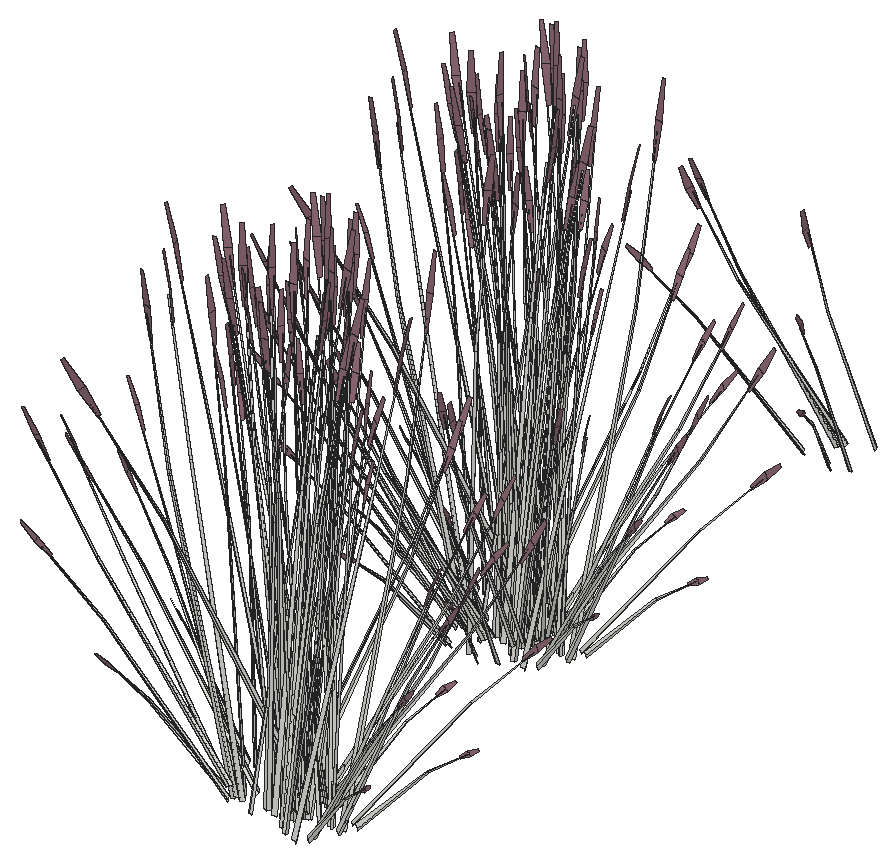
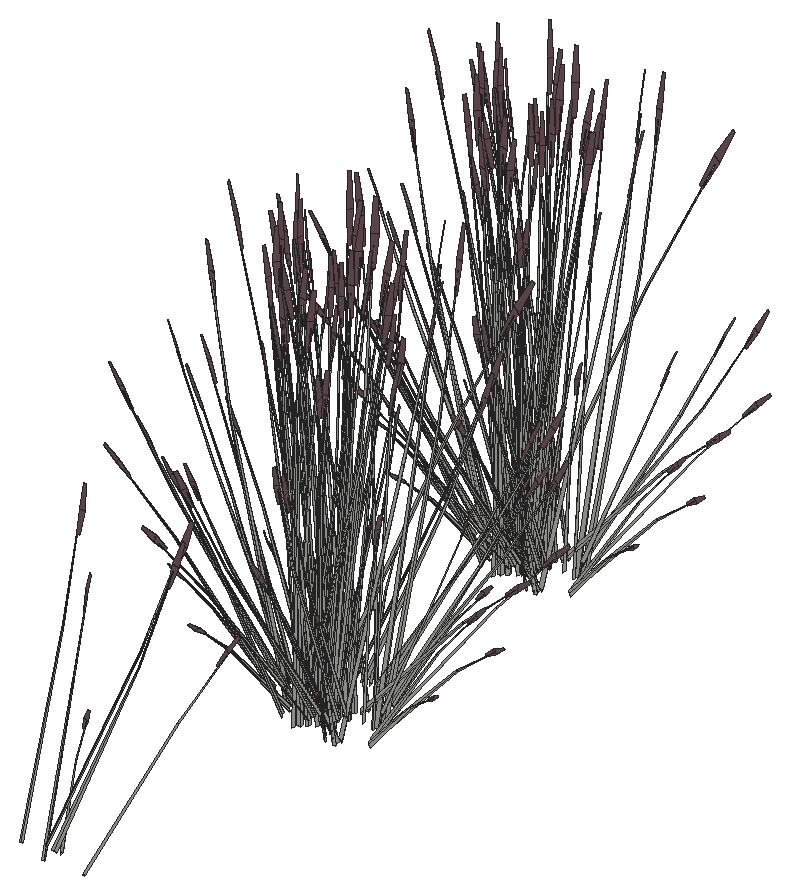
# SketchUp Ruby script. Lengths in inches.
U = 1.inch
M = Sketchup.active_model
def pt(a) = Geom::Point3d.new(a.map { |v| v * U })
def face(e, loops, mat)
  f = e.add_face(loops[0].map { |a| pt(a) })
  loops[1..].each { |l| e.add_face(l.map { |a| pt(a) }).erase! }
  f.material = f.back_material = mat if mat
  f
end
# faces: each face lists its corners as indices into pts; further lists are holes
def faces(e, pts, list, mat = nil) = list.each { |f| face(e, (f[0].is_a?(Array) ? f : [f]).map { |l| l.map { |i| pts[i] } }, mat) }
# xy, xz, yz: faces in a plane at the given z, y or x. An outline is a flat list of corners, or four numbers for a rectangle; further outlines are holes
def ring(l) = l.size == 4 ? [[l[0], l[1]], [l[2], l[1]], [l[2], l[3]], [l[0], l[3]]] : l.each_slice(2).to_a
def flat(e, list, mat, &to3) = list.each { |f| face(e, (f[0].is_a?(Array) ? f : [f]).map { |l| ring(l).map { |u, v| to3.(u, v) } }, mat) }
def xy(e, z, list, mat = nil) = flat(e, list, mat) { |x, y| [x, y, z] }
def xz(e, y, list, mat = nil) = flat(e, list, mat) { |x, z| [x, y, z] }
def yz(e, x, list, mat = nil) = flat(e, list, mat) { |y, z| [x, y, z] }
def lines(e, pts, list) = list.each { |a, b| e.add_line(pt(pts[a]), pt(pts[b])) }
# prism: a flat outline (further loops are holes) pulled along v
def prism(e, loops, v, mat = nil)
  f = face(e, loops, mat); d = Geom::Vector3d.new(v.map { |x| x * U })
  f.pushpull(f.normal.samedirection?(d) ? d.length : -d.length)
end
def box(e, o, s, mat = nil) = prism(e, [[o, [o[0] + s[0], o[1], o[2]], [o[0] + s[0], o[1] + s[1], o[2]], [o[0], o[1] + s[1], o[2]]]], [0, 0, s[2]], mat)
def at(x, y, z, deg = 0) = Geom::Transformation.translation(pt([x, y, z])) * Geom::Transformation.rotation(ORIGIN, Z_AXIS, deg.degrees)
def axes(o, x, y, z) = Geom::Transformation.new([*x, 0, *y, 0, *z, 0, *pt(o).to_a, 1])
def part(name) = M.definitions.add(name)
# library, detail: a bought-in or finely detailed component or shape, given as its bounding box
def library(name, o, s) = part(name).tap { |d| box(d.entities, o, s) }
def detail(e, o, s) = box(e.add_group.entities, o, s)
def put(e, d, t, mat = nil) = e.add_instance(d, t).tap { |i| i.material = mat if mat }
def group(e, t, mat = nil) = e.add_group.tap { |g| g.transformation = t; g.material = mat if mat }.entities
root = M.entities
M.materials.add("LightPink_Translucent").color = [144, 107, 117]
c1 = part("blade")
p = [[2.15,0.21,22],[0,0.17,0],[0.09,0.45,0],[2.18,0.31,22],[2.29,0.31,22],[0.38,0.45,0],
  [2.48,0.24,33],[2.49,0.24,33],[2.48,0.22,33]]
faces(c1.entities,p,[[0,1,2,3],[4,5,2,3],[6,3,4,7],[8,0,3,6]])
c2 = part("seeds")
p = [[0.3,-0.1,1.38],[-0.01,-0.03,1.59],[-0.01,-0.03,0.03],[0.14,-0.07,-0.07],[0.29,-0.03,3],[0.15,0.01,3.11]]
faces(c2.entities,p,[[0,1,2,3],[1,0,4,5]],"LightPink_Translucent")
c3 = part("blade with seeds")
put(c3.entities,c1,at(0,0,0))
put(c3.entities,c2,axes([2.4,0.25,30.99],[1.5799,-0.05474,1.17369],[-0.12525,1.92788,0.29478],[-0.07173,-0.02425,1.56792]))
put(root,c3,axes([53.92,557.8,45.33],[1.05902,0.41762,1.51261],[-1.03748,0.89969,0.59816],[-0.46471,-0.53324,1.26806]))
put(root,c3,axes([59,553.64,44.59],[-0.4378,-0.03068,1.43002],[-0.44851,-0.8229,-0.30754],[0.53783,-0.23279,0.61141]))
put(root,c3,axes([59.51,552.125,44.77],[-0.40819,0.5272,1.1486],[-0.35086,-0.70831,0.84392],[0.33713,-0.17749,0.25299]))
put(root,c3,axes([48.05,555.7,44.375],[-1.53239,0,0],[0,-1.1575,-0.51607],[0,-0.26363,1.63711]))
put(root,c3,axes([48.31,553.63,44.59],[0.23927,0.28834,1.43002],[-0.55135,0.78376,-0.30754],[-0.56612,-0.18733,0.61141]))
put(root,c3,axes([49.29,553.375,46.98],[-1.22504,-0.02494,-0.71045],[0.08228,-1.05005,0.08574],[-0.51899,-0.11081,1.00501]))
put(root,c3,axes([49.23,555.39,44.33],[-1.1399,0.87071,0.30756],[-1.1406,-0.86155,-0.36492],[-0.03981,-0.24727,1.64885]))
put(root,c3,axes([52.86,555.8,44.43],[1.3808,0.50196,0.24065],[-0.66454,1.04299,0.50002],[0,-0.24043,1.60543]))
put(root,c3,axes([48.89,553.59,46.68],[-0.88986,0.68603,-0.51099],[-0.77932,-0.72471,-0.3958],[-0.45212,-0.10438,0.97773]))
put(root,c3,axes([46.88,554.5,44.77],[0.78239,-0.07411,1.1486],[-0.49629,0.65296,0.84392],[-0.38663,-0.09795,0.25299]))
put(root,c3,axes([52.41,555.1,44.72],[-1.33077,0.06393,0.44739],[-0.12035,-1.06125,-0.21531],[0.23824,-0.10756,1.43643]))
put(root,c3,axes([48.98,555.875,44.48],[0,1.03566,0.49651],[-1.37109,0,0],[0,-0.23588,1.57504]))
put(root,c3,axes([58.6,556.1,46.68],[0.332,-0.94205,-0.51099],[1.13828,0.3229,-0.3958],[0.45829,-0.08638,0.97773]))
put(root,c3,axes([56.8,552.27,44.375],[0.7662,-1.03778,0],[1.28187,0.57875,-0.51607],[0.29196,0.13181,1.63711]))
put(root,c3,axes([52.36,555.48,44.36],[0.53281,1.15808,0.45755],[-1.52239,0.4027,0.17955],[0.01861,-0.2128,1.58856]))
put(root,c3,axes([59.82,556.37,43.98],[-0.7893,0.12429,1.41583],[-0.12563,-0.9893,0.08104],[0.55282,-0.14974,0.80566]))
put(root,c3,axes([52.1,556.39,44.72],[-0.59459,0.93321,0.44739],[-1.23546,-0.44912,-0.21531],[0,-0.21512,1.43643]))
put(root,c3,axes([54.28,555.58,44.21],[0,-1.19833,0],[1.53239,0,0],[0,0,1.79456]))
put(root,c3,axes([56.14,552.8125,44.48],[-1.14694,-0.51783,0.49651],[0.68554,-0.92854,0],[0.26122,0.11794,1.57504]))
put(root,c3,axes([58.38,556.45,46.98],[1.07686,-0.45739,-0.71045],[0.60013,0.94154,0.08574],[0.52031,-0.10696,1.00501]))
put(root,c3,axes([53.55,554.83,44.36],[-1.01611,0.93987,0.45755],[-1.20717,-0.82966,0.17955],[0.24496,-0.0938,1.58856]))
put(root,c3,axes([54.66,556.51,44.3],[-1.1399,-0.8914,-0.06131],[1.1406,-0.89194,0],[-0.03981,-0.03113,1.75571]))
put(root,c3,axes([51.79,553.28,44.47],[-0.35402,1.02926,0.17642],[-1.29548,-0.29127,0.35086],[0.22379,-0.00501,1.60407]))
put(root,c3,axes([54.5,554.42,44.62],[0.23642,-0.92427,0.1448],[1.15506,0.16044,-0.41347],[0.21021,0.09491,1.26744]))
put(root,c3,axes([52.5,556.62,44.36],[1.54892,0.2182,0.45755],[-0.31522,1.23236,0.17955],[-0.22636,-0.119,1.58856]))
put(root,c3,axes([54,554.67,44.72],[-0.73619,-0.86927,0.44739],[1.11511,-0.61213,-0.21531],[0.23824,0.10756,1.43643]))
put(root,c3,axes([51.67,558.59,44.47],[1.31687,-0.27488,0.17642],[0.32517,1.02297,0.35086],[-0.11745,-0.14905,1.60407]))
put(root,c3,axes([55.32,555.85,44.21],[1.37109,0,0],[0,1.07219,0],[0,0,1.78407]))
put(root,c3,axes([55.71,553.33,44.47],[-1.31687,0.27488,0.17642],[-0.32517,-1.02297,0.35086],[0.11745,0.14905,1.60407]))
put(root,c3,axes([54.88,555.3,44.38],[-1.54892,-0.2182,0.49198],[0.31522,-1.23236,0.19306],[0.22636,0.119,1.70813]))
put(root,c3,axes([53.64,558.34,44.2],[-0.39985,-0.89288,0],[1.1418,-0.31268,0],[0,0,1.54371]))
put(root,c3,axes([52.88,557.5,44.62],[-0.23642,0.92427,0.1448],[-1.15506,-0.16044,-0.41347],[-0.21021,-0.09491,1.26744]))
put(root,c3,axes([55.59,558.64,44.47],[0.35402,-1.02926,0.17642],[1.29548,0.29127,0.35086],[-0.22379,0.00501,1.60407]))
put(root,c3,axes([55.29,556.31,44.21],[0.85545,0.66896,0],[-0.85545,0.66896,0],[0,0,1.69266]))
put(root,c3,axes([50.43,555.05,45.34],[0.34834,-0.14982,1.77064],[0.12012,1.04605,0.13857],[-0.75452,0.1388,0.63284]))
put(root,c3,axes([57.61,556.02,44.47],[-0.96285,-0.75439,0.17642],[0.97031,-0.7317,0.35086],[-0.10634,0.15406,1.60407]))
put(root,c3,axes([61.46,556.71,44.77],[-0.75718,0.17097,1.1486],[0.35641,-0.70661,0.84392],[0.40168,0.04835,0.25299]))
put(root,c3,axes([53.36,558.75,44.2],[-1.23546,-0.46496,0],[0.59459,-0.96613,0],[0,0,1.62707]))
put(root,c3,axes([51.24,559.11,44.48],[1.14694,0.51783,0.49651],[-0.68554,0.92854,0],[-0.26122,-0.11794,1.57504]))
put(root,c3,axes([55.28,555.53,44.72],[0.59459,-0.93321,0.44739],[1.23546,0.44912,-0.21531],[0,0.21512,1.43643]))
put(root,c3,axes([55.05,556.06,44.29],[0,1.19774,-0.05637],[-1.53239,0,0],[0,0.03764,1.79368]))
put(root,c3,axes([48.02,555.62,46.68],[-0.332,0.94205,-0.51099],[-1.13828,-0.3229,-0.3958],[-0.45829,0.08638,0.97773]))
put(root,c3,axes([50.58,559.65,44.375],[-0.7662,1.03778,0],[-1.28187,-0.57875,-0.51607],[-0.29196,-0.13181,1.63711]))
put(root,c3,axes([58.4,556.05,44.48],[0,-1.03566,0.49651],[1.37109,0,0],[0,0.23588,1.57504]))
put(root,c3,axes([54.96,556.82,44.72],[1.33077,-0.06393,0.44739],[0.12035,1.06125,-0.21531],[-0.23824,0.10756,1.43643]))
put(root,c3,axes([55.8,555.74,44.62],[1.1418,-0.30203,0.1448],[0.39985,0.86246,-0.41347],[0,0.18981,1.26744]))
put(root,c3,axes([60.04,557.84,44.59],[-0.29514,-0.25472,1.43002],[0.38401,-0.84262,-0.30754],[0.59714,0.11414,0.61141]))
put(root,c3,axes([54.76,558.77,44.2],[1.23546,0.46496,0],[-0.59459,0.96613,0],[0,0,1.74954]))
put(root,c3,axes([55.26,559.8,44.19],[-0.75665,-1.04141,-0.05142],[1.28187,-0.57875,0.51607],[-0.31588,0.09915,1.6363]))
put(root,c3,axes([54.99,557.28,44.62],[0.90538,0.62224,0.1448],[-0.75521,0.70202,-0.41347],[-0.21021,0.09491,1.26744]))
put(root,c3,axes([57.33,558.35,46.98],[1.22504,0.02494,-0.71045],[-0.08228,1.05005,0.08574],[0.51899,0.11081,1.00501]))
put(root,c3,axes([55.95,559.19,44.48],[1.14694,-0.51783,0.49651],[0.68554,0.92854,0],[-0.26122,0.11794,1.57504]))
put(root,c3,axes([54.32,558.375,44.29],[0.53281,1.18979,-0.06012],[-1.52239,0.41691,0],[0.01861,0.04155,1.72173]))
put(root,c3,axes([46.66,557.83,44.59],[0.42589,0.08502,1.43002],[0.2745,0.86839,-0.30754],[-0.57851,0.16255,0.61141]))
put(root,c3,axes([59.33,556.22,44.375],[1.53239,0,0],[0,1.1575,-0.51607],[0,0.26363,1.63711]))
put(root,c3,axes([58.72,556.82,44.2],[-1.53164,-0.00828,-0.04976],[0,-1.1575,0.49943],[-0.04813,0.2635,1.58352]))
put(root,c3,axes([45.77,559.65,44.77],[0.51072,-0.46938,1.1486],[0.20153,0.74307,0.84392],[-0.36908,0.13305,0.25299]))
put(root,c3,axes([55.29,559.26,44.33],[1.53422,0.33662,0.30756],[-0.38383,1.20322,-0.36492],[-0.25393,0.15059,1.64885]))
put(root,c3,axes([57.25,559.16,44.77],[-0.69001,-0.29779,1.1486],[0.89096,-0.30257,0.84392],[0.24031,0.2563,0.25299]))
put(root,c3,axes([48.58,557.72,46.68],[0.31482,0.94565,-0.51099],[-1.19224,0.16542,-0.3958],[-0.34166,0.254,0.97773]))
put(root,c3,axes([56.22,559.91,44.375],[0.7662,1.03778,0],[-1.28187,0.57875,-0.51607],[-0.29196,0.13181,1.63711]))
put(root,c3,axes([55.57,555.8,44.84],[-0.03348,-0.97511,1.41272],[1.51511,0.25277,0.59816],[-0.35835,0.53357,1.3335]))
put(root,c3,axes([55.6875,559.57,46.68],[1.20928,-0.24619,-0.51099],[0.21154,0.93233,-0.3958],[0.32481,0.26718,0.97773]))
put(root,c3,axes([57.36,560.51,44.67],[-0.78586,-0.03248,1.0506],[0.51898,-0.68985,0.58006],[0.31045,0.24509,0.8241]))
put(root,c3,axes([54.79,558.84,44.59],[0.02163,-0.34331,1.43002],[1.03345,-0.38348,-0.30754],[0.31903,0.4109,0.61141]))
put(root,c3,axes([50.1,561.7,44.77],[-0.03171,-0.6158,1.1486],[0.7925,0.43922,0.84392],[-0.15586,0.29352,0.25299]))
put(root,c3,axes([50.4,559.32,47],[0.87728,0.69587,-0.5672],[-0.92674,0.60943,-0.43934],[-0.13348,0.35356,1.08528]))
put(root,c3,axes([49.45,560.37,44.82],[1.11329,-0.1834,0.06507],[0.25594,0.73887,-0.86304],[-0.07058,0.37403,0.7736]))
put(root,c3,axes([53,560,46.68],[1.20468,0.25962,-0.51099],[-0.41292,0.89013,-0.3958],[0.11046,0.35838,0.97773]))
put(root,c3,axes([50.13,559.01,47.34],[-0.03189,0.95798,-0.7886],[-1.34277,-0.06434,0.09517],[-0.14171,0.40585,1.11556]))
put(root,c3,axes([52.5625,559.83,46.98],[0.5849,0.8421,-0.71045],[-1.20401,0.4693,0.08574],[0.13677,0.40688,1.00501]))
put(root,c3,axes([49.18,561.15,44.59],[0.38672,-0.16338,1.43002],[0.95481,0.49262,-0.30754],[-0.28419,0.42626,0.61141]))
put(root,c3,axes([49.68,560.35,45.36],[0.02693,-0.53464,1.54345],[1.21102,0.2824,0.21329],[-0.10493,0.5698,0.72882]))
put(root,c3,axes([51.82,589.99,44.59],[-0.34835,0.20963,1.43002],[-1.04325,-0.36691,-0.30754],[0.19338,-0.4563,0.61141]))
put(root,c3,axes([50.23,590.72,46.98],[-0.5849,-0.8421,-0.71045],[1.20401,-0.4693,0.08574],[-0.13677,-0.40688,1.00501]))
put(root,c3,axes([46.42,589.6,44.59],[-0.07421,0.33879,1.43002],[-1.08488,0.28361,-0.30754],[-0.25359,-0.4379,0.61141]))
put(root,c3,axes([52.66,591.55,46.98],[0.03189,-0.95798,-0.71045],[1.34277,0.06434,0.08574],[0.14171,-0.40585,1.00501]))
put(root,c3,axes([49.79,590.55,46.68],[-1.20468,-0.25962,-0.51099],[0.41292,-0.89013,-0.3958],[-0.11046,-0.35838,0.97773]))
put(root,c3,axes([50.54,588.33,44.77],[0.15721,0.60392,1.1486],[-0.87211,-0.33448,0.84392],[0.09385,-0.30923,0.25299]))
put(root,c3,axes([52.39,591.23,46.68],[-0.87728,-0.69587,-0.51099],[0.92674,-0.60943,-0.3958],[0.13348,-0.35356,0.97773]))
put(root,c3,axes([46.05,589.05,44.77],[0.63926,0.36046,1.1486],[-0.93099,0.21668,0.84392],[-0.1992,-0.27702,0.25299]))
put(root,c3,axes([47.59,590.96,46.98],[-1.04497,-0.50058,-0.71045],[0.74264,-0.8772,0.08574],[-0.3786,-0.29889,1.00501]))
put(root,c3,axes([47.11,590.99,46.68],[-1.20928,0.24619,-0.51099],[-0.21154,-0.93233,-0.3958],[-0.32481,-0.26718,0.97773]))
put(root,c3,axes([54.25,593.21,46.98],[0.64013,-0.81717,-0.71045],[1.12174,0.58074,0.08574],[0.38221,-0.29607,1.00501]))
put(root,c3,axes([47.33,590.83,44.375],[-0.7662,-1.03778,0],[1.28187,-0.57875,-0.51607],[0.29196,-0.13181,1.63711]))
put(root,c3,axes([54.22,592.83,46.68],[-0.31482,-0.94565,-0.51099],[1.19224,-0.16542,-0.3958],[0.34166,-0.254,0.97773]))
put(root,c3,axes([50.09,596.625,45.33],[1.05902,0.41762,1.51261],[-1.03748,0.89969,0.59816],[-0.46471,-0.53324,1.26806]))
put(root,c3,axes([55.17,592.46,44.59],[-0.4378,-0.03068,1.43002],[-0.44851,-0.8229,-0.30754],[0.53783,-0.23279,0.61141]))
put(root,c3,axes([55.68,590.95,44.77],[-0.40819,0.5272,1.1486],[-0.35086,-0.70831,0.84392],[0.33713,-0.17749,0.25299]))
put(root,c3,axes([44.22,594.52,44.375],[-1.53239,0,0],[0,-1.1575,-0.51607],[0,-0.26363,1.63711]))
put(root,c3,axes([44.48,592.46,44.59],[0.23927,0.28834,1.43002],[-0.55135,0.78376,-0.30754],[-0.56612,-0.18733,0.61141]))
put(root,c3,axes([45.46,592.2,46.98],[-1.22504,-0.02494,-0.71045],[0.08228,-1.05005,0.08574],[-0.51899,-0.11081,1.00501]))
put(root,c3,axes([45.4,594.22,44.33],[-1.1399,0.87071,0.30756],[-1.1406,-0.86155,-0.36492],[-0.03981,-0.24727,1.64885]))
put(root,c3,axes([49.03,594.625,44.43],[1.3808,0.50196,0.24065],[-0.66454,1.04299,0.50002],[0,-0.24043,1.60543]))
put(root,c3,axes([45.06,592.41,46.68],[-0.88986,0.68603,-0.51099],[-0.77932,-0.72471,-0.3958],[-0.45212,-0.10438,0.97773]))
put(root,c3,axes([43.05,593.32,44.77],[0.78239,-0.07411,1.1486],[-0.49629,0.65296,0.84392],[-0.38663,-0.09795,0.25299]))
put(root,c3,axes([48.58,593.93,44.72],[-1.33077,0.06393,0.44739],[-0.12035,-1.06125,-0.21531],[0.23824,-0.10756,1.43643]))
put(root,c3,axes([45.15,594.7,44.48],[0,1.03566,0.49651],[-1.37109,0,0],[0,-0.23588,1.57504]))
put(root,c3,axes([54.77,594.93,46.68],[0.332,-0.94205,-0.51099],[1.13828,0.3229,-0.3958],[0.45829,-0.08638,0.97773]))
put(root,c3,axes([52.97,591.09,44.375],[0.7662,-1.03778,0],[1.28187,0.57875,-0.51607],[0.29196,0.13181,1.63711]))
put(root,c3,axes([48.53,594.31,44.36],[0.53281,1.15808,0.45755],[-1.52239,0.4027,0.17955],[0.01861,-0.2128,1.58856]))
put(root,c3,axes([55.99,595.2,43.98],[-0.7893,0.12429,1.41583],[-0.12563,-0.9893,0.08104],[0.55282,-0.14974,0.80566]))
put(root,c3,axes([48.27,595.22,44.72],[-0.59459,0.93321,0.44739],[-1.23546,-0.44912,-0.21531],[0,-0.21512,1.43643]))
put(root,c3,axes([50.45,594.41,44.21],[0,-1.19833,0],[1.53239,0,0],[0,0,1.79456]))
put(root,c3,axes([52.31,591.64,44.48],[-1.14694,-0.51783,0.49651],[0.68554,-0.92854,0],[0.26122,0.11794,1.57504]))
put(root,c3,axes([54.55,595.27,46.98],[1.07686,-0.45739,-0.71045],[0.60013,0.94154,0.08574],[0.52031,-0.10696,1.00501]))
put(root,c3,axes([49.72,593.65,44.36],[-1.01611,0.93987,0.45755],[-1.20717,-0.82966,0.17955],[0.24496,-0.0938,1.58856]))
put(root,c3,axes([50.83,595.33,44.3],[-1.1399,-0.8914,-0.06131],[1.1406,-0.89194,0],[-0.03981,-0.03113,1.75571]))
put(root,c3,axes([47.96,592.1,44.47],[-0.35402,1.02926,0.17642],[-1.29548,-0.29127,0.35086],[0.22379,-0.00501,1.60407]))
put(root,c3,axes([50.67,593.25,44.62],[0.23642,-0.92427,0.1448],[1.15506,0.16044,-0.41347],[0.21021,0.09491,1.26744]))
put(root,c3,axes([48.67,595.44,44.36],[1.54892,0.2182,0.45755],[-0.31522,1.23236,0.17955],[-0.22636,-0.119,1.58856]))
put(root,c3,axes([50.17,593.49,44.72],[-0.73619,-0.86927,0.44739],[1.11511,-0.61213,-0.21531],[0.23824,0.10756,1.43643]))
put(root,c3,axes([47.84,597.41,44.47],[1.31687,-0.27488,0.17642],[0.32517,1.02297,0.35086],[-0.11745,-0.14905,1.60407]))
put(root,c3,axes([51.49,594.67,44.21],[1.37109,0,0],[0,1.07219,0],[0,0,1.78407]))
put(root,c3,axes([51.88,592.16,44.47],[-1.31687,0.27488,0.17642],[-0.32517,-1.02297,0.35086],[0.11745,0.14905,1.60407]))
put(root,c3,axes([51.05,594.13,44.38],[-1.54892,-0.2182,0.49198],[0.31522,-1.23236,0.19306],[0.22636,0.119,1.70813]))
put(root,c3,axes([49.8125,597.17,44.2],[-0.39985,-0.89288,0],[1.1418,-0.31268,0],[0,0,1.54371]))
put(root,c3,axes([49.05,596.32,44.62],[-0.23642,0.92427,0.1448],[-1.15506,-0.16044,-0.41347],[-0.21021,-0.09491,1.26744]))
put(root,c3,axes([51.76,597.47,44.47],[0.35402,-1.02926,0.17642],[1.29548,0.29127,0.35086],[-0.22379,0.00501,1.60407]))
put(root,c3,axes([51.46,595.13,44.21],[0.85545,0.66896,0],[-0.85545,0.66896,0],[0,0,1.69266]))
put(root,c3,axes([46.6,593.88,45.34],[0.34834,-0.14982,1.77064],[0.12012,1.04605,0.13857],[-0.75452,0.1388,0.63284]))
put(root,c3,axes([53.78,594.84,44.47],[-0.96285,-0.75439,0.17642],[0.97031,-0.7317,0.35086],[-0.10634,0.15406,1.60407]))
put(root,c3,axes([57.63,595.53,44.77],[-0.75718,0.17097,1.1486],[0.35641,-0.70661,0.84392],[0.40168,0.04835,0.25299]))
put(root,c3,axes([49.53,597.57,44.2],[-1.23546,-0.46496,0],[0.59459,-0.96613,0],[0,0,1.62707]))
put(root,c3,axes([47.41,597.93,44.48],[1.14694,0.51783,0.49651],[-0.68554,0.92854,0],[-0.26122,-0.11794,1.57504]))
put(root,c3,axes([51.45,594.35,44.72],[0.59459,-0.93321,0.44739],[1.23546,0.44912,-0.21531],[0,0.21512,1.43643]))
put(root,c3,axes([51.22,594.88,44.29],[0,1.19774,-0.05637],[-1.53239,0,0],[0,0.03764,1.79368]))
put(root,c3,axes([44.19,594.45,46.68],[-0.332,0.94205,-0.51099],[-1.13828,-0.3229,-0.3958],[-0.45829,0.08638,0.97773]))
put(root,c3,axes([46.75,598.48,44.375],[-0.7662,1.03778,0],[-1.28187,-0.57875,-0.51607],[-0.29196,-0.13181,1.63711]))
put(root,c3,axes([54.57,594.87,44.48],[0,-1.03566,0.49651],[1.37109,0,0],[0,0.23588,1.57504]))
put(root,c3,axes([51.13,595.65,44.72],[1.33077,-0.06393,0.44739],[0.12035,1.06125,-0.21531],[-0.23824,0.10756,1.43643]))
put(root,c3,axes([51.97,594.5625,44.62],[1.1418,-0.30203,0.1448],[0.39985,0.86246,-0.41347],[0,0.18981,1.26744]))
put(root,c3,axes([56.21,596.67,44.59],[-0.29514,-0.25472,1.43002],[0.38401,-0.84262,-0.30754],[0.59714,0.11414,0.61141]))
put(root,c3,axes([50.93,597.59,44.2],[1.23546,0.46496,0],[-0.59459,0.96613,0],[0,0,1.74954]))
put(root,c3,axes([51.43,598.62,44.19],[-0.75665,-1.04141,-0.05142],[1.28187,-0.57875,0.51607],[-0.31588,0.09915,1.6363]))
put(root,c3,axes([51.16,596.1,44.62],[0.90538,0.62224,0.1448],[-0.75521,0.70202,-0.41347],[-0.21021,0.09491,1.26744]))
put(root,c3,axes([53.5,597.18,46.98],[1.22504,0.02494,-0.71045],[-0.08228,1.05005,0.08574],[0.51899,0.11081,1.00501]))
put(root,c3,axes([52.12,598.02,44.48],[1.14694,-0.51783,0.49651],[0.68554,0.92854,0],[-0.26122,0.11794,1.57504]))
put(root,c3,axes([50.49,597.2,44.29],[0.53281,1.18979,-0.06012],[-1.52239,0.41691,0],[0.01861,0.04155,1.72173]))
put(root,c3,axes([42.83,596.66,44.59],[0.42589,0.08502,1.43002],[0.2745,0.86839,-0.30754],[-0.57851,0.16255,0.61141]))
put(root,c3,axes([55.5,595.05,44.375],[1.53239,0,0],[0,1.1575,-0.51607],[0,0.26363,1.63711]))
put(root,c3,axes([54.89,595.64,44.2],[-1.53164,-0.00828,-0.04976],[0,-1.1575,0.49943],[-0.04813,0.2635,1.58352]))
put(root,c3,axes([41.94,598.48,44.77],[0.51072,-0.46938,1.1486],[0.20153,0.74307,0.84392],[-0.36908,0.13305,0.25299]))
put(root,c3,axes([51.46,598.09,44.33],[1.53422,0.33662,0.30756],[-0.38383,1.20322,-0.36492],[-0.25393,0.15059,1.64885]))
put(root,c3,axes([53.42,597.98,44.77],[-0.69001,-0.29779,1.1486],[0.89096,-0.30257,0.84392],[0.24031,0.2563,0.25299]))
put(root,c3,axes([44.75,596.55,46.68],[0.31482,0.94565,-0.51099],[-1.19224,0.16542,-0.3958],[-0.34166,0.254,0.97773]))
put(root,c3,axes([52.39,598.74,44.375],[0.7662,1.03778,0],[-1.28187,0.57875,-0.51607],[-0.29196,0.13181,1.63711]))
put(root,c3,axes([51.74,594.63,44.84],[-0.03348,-0.97511,1.41272],[1.51511,0.25277,0.59816],[-0.35835,0.53357,1.3335]))
put(root,c3,axes([51.86,598.39,46.68],[1.20928,-0.24619,-0.51099],[0.21154,0.93233,-0.3958],[0.32481,0.26718,0.97773]))
put(root,c3,axes([53.53,599.34,44.67],[-0.78586,-0.03248,1.0506],[0.51898,-0.68985,0.58006],[0.31045,0.24509,0.8241]))
put(root,c3,axes([50.96,597.66,44.59],[0.02163,-0.34331,1.43002],[1.03345,-0.38348,-0.30754],[0.31903,0.4109,0.61141]))
put(root,c3,axes([46.27,600.53,44.77],[-0.03171,-0.6158,1.1486],[0.7925,0.43922,0.84392],[-0.15586,0.29352,0.25299]))
put(root,c3,axes([46.57,598.15,47],[0.87728,0.69587,-0.5672],[-0.92674,0.60943,-0.43934],[-0.13348,0.35356,1.08528]))
put(root,c3,axes([45.62,599.19,44.82],[1.11329,-0.1834,0.06507],[0.25594,0.73887,-0.86304],[-0.07058,0.37403,0.7736]))
put(root,c3,axes([49.17,598.82,46.68],[1.20468,0.25962,-0.51099],[-0.41292,0.89013,-0.3958],[0.11046,0.35838,0.97773]))
put(root,c3,axes([46.3,597.83,47.34],[-0.03189,0.95798,-0.7886],[-1.34277,-0.06434,0.09517],[-0.14171,0.40585,1.11556]))
put(root,c3,axes([48.73,598.65,46.98],[0.5849,0.8421,-0.71045],[-1.20401,0.4693,0.08574],[0.13677,0.40688,1.00501]))
put(root,c3,axes([45.35,599.98,44.59],[0.38672,-0.16338,1.43002],[0.95481,0.49262,-0.30754],[-0.28419,0.42626,0.61141]))
put(root,c3,axes([45.85,599.18,45.36],[0.02693,-0.53464,1.54345],[1.21102,0.2824,0.21329],[-0.10493,0.5698,0.72882]))
put(root,c3,axes([54.61,639,44.59],[-0.34835,0.20963,1.43002],[-1.04325,-0.36691,-0.30754],[0.19338,-0.4563,0.61141]))
put(root,c3,axes([53.02,639.73,46.98],[-0.5849,-0.8421,-0.71045],[1.20401,-0.4693,0.08574],[-0.13677,-0.40688,1.00501]))
put(root,c3,axes([49.22,638.61,44.59],[-0.07421,0.33879,1.43002],[-1.08488,0.28361,-0.30754],[-0.25359,-0.4379,0.61141]))
put(root,c3,axes([55.46,640.56,46.98],[0.03189,-0.95798,-0.71045],[1.34277,0.06434,0.08574],[0.14171,-0.40585,1.00501]))
put(root,c3,axes([52.58,639.5625,46.68],[-1.20468,-0.25962,-0.51099],[0.41292,-0.89013,-0.3958],[-0.11046,-0.35838,0.97773]))
put(root,c3,axes([53.33,637.34,44.77],[0.15721,0.60392,1.1486],[-0.87211,-0.33448,0.84392],[0.09385,-0.30923,0.25299]))
